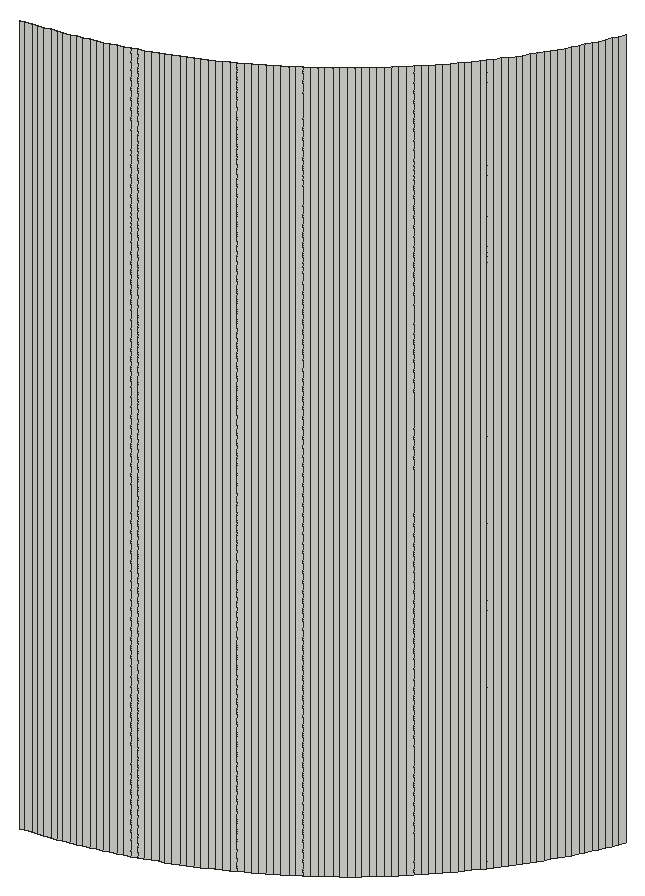
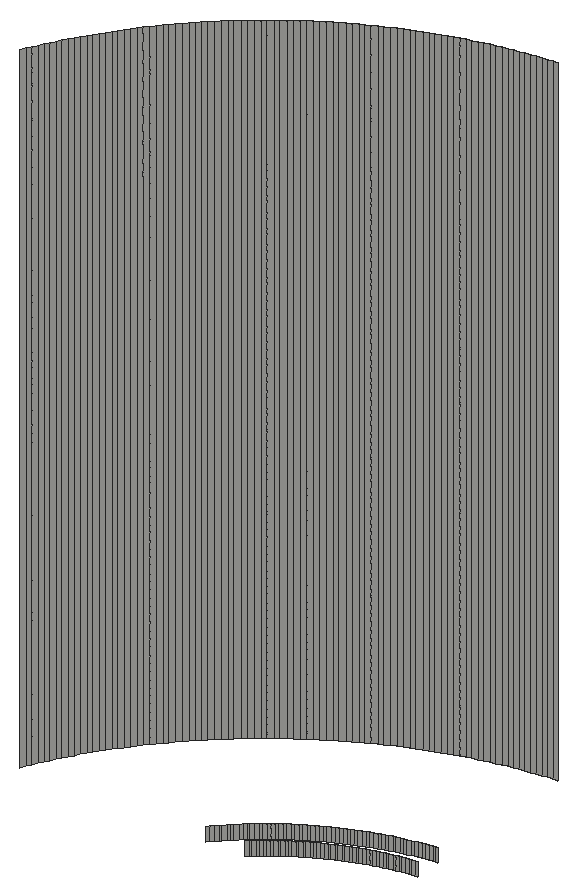
# SketchUp Ruby script. Lengths in inches.
U = 1.inch
M = Sketchup.active_model
def pt(a) = Geom::Point3d.new(a.map { |v| v * U })
def face(e, loops, mat)
  f = e.add_face(loops[0].map { |a| pt(a) })
  loops[1..].each { |l| e.add_face(l.map { |a| pt(a) }).erase! }
  f.material = f.back_material = mat if mat
  f
end
# faces: each face lists its corners as indices into pts; further lists are holes
def faces(e, pts, list, mat = nil) = list.each { |f| face(e, (f[0].is_a?(Array) ? f : [f]).map { |l| l.map { |i| pts[i] } }, mat) }
# xy, xz, yz: faces in a plane at the given z, y or x. An outline is a flat list of corners, or four numbers for a rectangle; further outlines are holes
def ring(l) = l.size == 4 ? [[l[0], l[1]], [l[2], l[1]], [l[2], l[3]], [l[0], l[3]]] : l.each_slice(2).to_a
def flat(e, list, mat, &to3) = list.each { |f| face(e, (f[0].is_a?(Array) ? f : [f]).map { |l| ring(l).map { |u, v| to3.(u, v) } }, mat) }
def xy(e, z, list, mat = nil) = flat(e, list, mat) { |x, y| [x, y, z] }
def xz(e, y, list, mat = nil) = flat(e, list, mat) { |x, z| [x, y, z] }
def yz(e, x, list, mat = nil) = flat(e, list, mat) { |y, z| [x, y, z] }
def lines(e, pts, list) = list.each { |a, b| e.add_line(pt(pts[a]), pt(pts[b])) }
# prism: a flat outline (further loops are holes) pulled along v
def prism(e, loops, v, mat = nil)
  f = face(e, loops, mat); d = Geom::Vector3d.new(v.map { |x| x * U })
  f.pushpull(f.normal.samedirection?(d) ? d.length : -d.length)
end
def box(e, o, s, mat = nil) = prism(e, [[o, [o[0] + s[0], o[1], o[2]], [o[0] + s[0], o[1] + s[1], o[2]], [o[0], o[1] + s[1], o[2]]]], [0, 0, s[2]], mat)
def at(x, y, z, deg = 0) = Geom::Transformation.translation(pt([x, y, z])) * Geom::Transformation.rotation(ORIGIN, Z_AXIS, deg.degrees)
def axes(o, x, y, z) = Geom::Transformation.new([*x, 0, *y, 0, *z, 0, *pt(o).to_a, 1])
def part(name) = M.definitions.add(name)
# library, detail: a bought-in or finely detailed component or shape, given as its bounding box
def library(name, o, s) = part(name).tap { |d| box(d.entities, o, s) }
def detail(e, o, s) = box(e.add_group.entities, o, s)
def put(e, d, t, mat = nil) = e.add_instance(d, t).tap { |i| i.material = mat if mat }
def group(e, t, mat = nil) = e.add_group.tap { |g| g.transformation = t; g.material = mat if mat }.entities
root = M.entities
p = [[368.95,214,228],[369.1,214.01,228],[369.1,214.01,252],[368.95,214,252],[369.29,214.04,228],[369.29,214.04,252],
  [369.48,214.0625,228],[369.48,214.0625,252],[369.67,214.09,228],[369.67,214.09,252],[369.85,214.12,228],[369.85,214.12,252],
  [370.04,214.15,228],[370.04,214.15,252],[370.23,214.18,228],[370.23,214.18,252],[370.42,214.22,228],[370.42,214.22,252],
  [370.61,214.25,228],[370.61,214.25,252],[370.8,214.29,228],[370.8,214.29,252],[370.98,214.34,228],[370.98,214.34,252],
  [371.17,214.38,228],[371.17,214.38,252],[371.35,214.43,228],[371.35,214.43,252],[371.54,214.48,228],[371.54,214.48,252],
  [371.72,214.53,228],[371.72,214.53,252],[371.91,214.58,228],[371.91,214.58,252],[372.09,214.64,228],[372.09,214.64,252],
  [372.27,214.7,228],[372.27,214.7,252],[372.45,214.76,228],[372.45,214.76,252],[372.64,214.82,228],[372.64,214.82,252],
  [372.82,214.89,228],[372.82,214.89,252],[372.99,214.95,228],[372.99,214.95,252],[373.17,215.02,228],[373.17,215.02,252],
  [373.35,215.1,228],[373.35,215.1,252],[373.53,215.17,228],[373.53,215.17,252],[373.7,215.25,228],[373.7,215.25,252],
  [373.88,215.32,228],[373.88,215.32,252],[374.05,215.41,228],[374.05,215.41,252],[374.22,215.49,228],[374.22,215.49,252],
  [374.4,215.57,228],[374.4,215.57,252],[374.57,215.66,228],[374.57,215.66,252],[374.74,215.75,228],[374.74,215.75,252],
  [374.91,215.84,228],[374.91,215.84,252],[375.07,215.93,228],[375.07,215.93,252],[375.24,216.03,228],[375.24,216.03,252],
  [375.4,216.125,228],[375.4,216.125,252],[375.57,216.22,228],[375.57,216.22,252],[375.73,216.32,228],[375.73,216.32,252],
  [375.89,216.43,228],[375.89,216.43,252],[376.05,216.53,228],[376.05,216.53,252],[376.21,216.64,228],[376.21,216.64,252],
  [376.37,216.75,228],[376.37,216.75,252],[376.52,216.86,228],[376.52,216.86,252],[376.68,216.97,228],[376.68,216.97,252],
  [376.83,217.09,228],[376.83,217.09,252],[376.98,217.2,228],[376.98,217.2,252],[377.13,217.32,228],[377.13,217.32,252],
  [377.28,217.44,228],[377.28,217.44,252],[377.43,217.56,228],[377.43,217.56,252],[377.58,217.6875,228],[377.58,217.6875,252],
  [377.72,217.8125,228],[377.72,217.8125,252],[377.86,217.94,228],[377.86,217.94,252],[378.01,218.07,228],[378.01,218.07,252],
  [378.15,218.2,228],[378.15,218.2,252],[378.28,218.33,228],[378.28,218.33,252],[378.42,218.47,228],[378.42,218.47,252],
  [378.56,218.61,228],[378.56,218.61,252],[378.6875,218.74,228],[378.6875,218.74,252],[378.82,218.88,228],[378.82,218.88,252],
  [378.95,219.02,228],[378.95,219.02,252],[379.08,219.17,228],[379.08,219.17,252],[379.2,219.31,228],[379.2,219.31,252],
  [379.33,219.46,228],[379.33,219.46,252],[379.45,219.6,228],[379.45,219.6,252],[379.57,219.75,228],[379.57,219.75,252],
  [379.69,219.9,228],[379.69,219.9,252],[379.81,220.05,228],[379.81,220.05,252],[368.6875,220.01,228],[368.62,220,228],
  [368.62,220,228.5],[368.6875,220.01,228.5],[368.8,220.02,228],[368.8,220.02,228.5],[368.92,220.04,228],[368.92,220.04,228.5],
  [369.03,220.0625,228],[369.03,220.0625,228.5],[369.15,220.08,228],[369.15,220.08,228.5],[369.27,220.1,228],[369.27,220.1,228.5],
  [369.38,220.13,228],[369.38,220.13,228.5],[369.5,220.15,228],[369.5,220.15,228.5],[379.92,220.21,228],[379.92,220.21,252],
  [369.61,220.18,228],[369.61,220.18,228.5],[369.73,220.21,228],[369.73,220.21,228.5],[369.84,220.23,228],[369.84,220.23,228.5],
  [369.95,220.27,228],[369.95,220.27,228.5],[380.04,220.36,228],[380.04,220.36,252],[370.07,220.3,228],[370.07,220.3,228.5],
  [370.18,220.33,228],[370.18,220.33,228.5],[370.29,220.36,228],[370.29,220.36,228.5],[370.41,220.4,228],[370.41,220.4,228.5],
  [370.52,220.4375,228],[370.52,220.4375,228.5],[370.63,220.48,228],[370.63,220.48,228.5],[380.15,220.52,228],[380.15,220.52,252],
  [370.74,220.52,228],[370.74,220.52,228.5],[370.85,220.56,228],[370.85,220.56,228.5],[380.26,220.67,228],[380.26,220.67,252],
  [370.96,220.6,228],[370.96,220.6,228.5],[371.07,220.65,228],[371.07,220.65,228.5],[371.18,220.69,228],[371.18,220.69,228.5],
  [371.28,220.74,228],[371.28,220.74,228.5],[371.39,220.79,228],[371.39,220.79,228.5],[380.36,220.83,228],[380.36,220.83,252],
  [371.5,220.84,228],[371.5,220.84,228.5],[371.61,220.89,228],[371.61,220.89,228.5],[380.47,220.99,228],[380.47,220.99,252],
  [371.71,220.9375,228],[371.71,220.9375,228.5],[371.82,220.99,228],[371.82,220.99,228.5],[368.56,221,228],[368.66,221.01,228],
  [368.66,221.01,228.5],[368.56,221,228.5],[368.76,221.03,228],[368.76,221.03,228.5],[368.87,221.05,228],[368.87,221.05,228.5],
  [368.97,221.07,228],[368.97,221.07,228.5],[371.92,221.05,228],[371.92,221.05,228.5],[372.02,221.1,228],[372.02,221.1,228.5],
  [380.57,221.15,228],[380.57,221.15,252],[369.07,221.09,228],[369.07,221.09,228.5],[369.18,221.11,228],[369.18,221.11,228.5],
  [369.28,221.13,228],[369.28,221.13,228.5],[369.38,221.15,228],[369.38,221.15,228.5],[372.125,221.16,228],[372.125,221.16,228.5],
  [369.49,221.18,228],[369.49,221.18,228.5],[369.59,221.2,228],[369.59,221.2,228.5],[369.69,221.23,228],[369.69,221.23,228.5],
  [369.79,221.26,228],[369.79,221.26,228.5],[372.23,221.22,228],[372.23,221.22,228.5],[372.33,221.28,228],[372.33,221.28,228.5],
  [380.68,221.31,228],[380.68,221.31,252],[369.89,221.29,228],[369.89,221.29,228.5],[369.99,221.32,228],[369.99,221.32,228.5],
  [370.09,221.35,228],[370.09,221.35,228.5],[372.43,221.34,228],[372.43,221.34,228.5],[372.53,221.4,228],[372.53,221.4,228.5],
  [380.78,221.48,228],[380.78,221.48,252],[370.19,221.38,228],[370.19,221.38,228.5],[370.29,221.42,228],[370.29,221.42,228.5],
  [370.39,221.46,228],[370.39,221.46,228.5],[372.63,221.46,228],[372.63,221.46,228.5],[370.49,221.49,228],[370.49,221.49,228.5],
  [370.59,221.53,228],[370.59,221.53,228.5],[370.6875,221.57,228],[370.6875,221.57,228.5],[372.73,221.53,228],[372.73,221.53,228.5],
  [372.83,221.59,228],[372.83,221.59,228.5],[380.87,221.64,228],[380.87,221.64,252],[370.78,221.61,228],[370.78,221.61,228.5],
  [370.88,221.65,228],[370.88,221.65,228.5],[372.92,221.66,228],[372.92,221.66,228.5],[380.97,221.81,228],[380.97,221.81,252],
  [370.98,221.7,228],[370.98,221.7,228.5],[371.07,221.74,228],[371.07,221.74,228.5],[371.17,221.79,228],[371.17,221.79,228.5],
  [373.02,221.73,228],[373.02,221.73,228.5],[373.11,221.8,228],[373.11,221.8,228.5],[371.26,221.83,228],[371.26,221.83,228.5],
  [371.36,221.88,228],[371.36,221.88,228.5],[373.21,221.87,228],[373.21,221.87,228.5],[381.0625,221.98,228],[381.0625,221.98,252],
  [371.45,221.93,228],[371.45,221.93,228.5],[371.54,221.98,228],[371.54,221.98,228.5],[373.3,221.94,228],[373.3,221.94,228.5],
  [373.39,222.01,228],[373.39,222.01,228.5],[371.64,222.03,228],[371.64,222.03,228.5],[371.73,222.08,228],[371.73,222.08,228.5],
  [373.49,222.09,228],[373.49,222.09,228.5],[381.15,222.14,228],[381.15,222.14,252],[371.82,222.14,228],[371.82,222.14,228.5],
  [371.91,222.19,228],[371.91,222.19,228.5],[373.58,222.16,228],[373.58,222.16,228.5],[381.24,222.3125,228],[381.24,222.3125,252],
  [372,222.25,228],[372,222.25,228.5],[372.09,222.3,228],[372.09,222.3,228.5],[373.67,222.24,228],[373.67,222.24,228.5],
  [373.76,222.32,228],[373.76,222.32,228.5],[372.17,222.36,228],[372.17,222.36,228.5],[373.84,222.39,228],[373.84,222.39,228.5],
  [381.33,222.48,228],[381.33,222.48,252],[372.26,222.42,228],[372.26,222.42,228.5],[372.35,222.48,228],[372.35,222.48,228.5],
  [373.93,222.47,228],[373.93,222.47,228.5],[372.43,222.54,228],[372.43,222.54,228.5],[372.52,222.6,228],[372.52,222.6,228.5],
  [374.02,222.55,228],[374.02,222.55,228.5],[381.42,222.66,228],[381.42,222.66,252],[372.6,222.67,228],[372.6,222.67,228.5],
  [374.1,222.64,228],[374.1,222.64,228.5],[374.18,222.72,228],[374.18,222.72,228.5],[372.6875,222.73,228],[372.6875,222.73,228.5],
  [372.77,222.8,228],[372.77,222.8,228.5],[374.27,222.8,228],[374.27,222.8,228.5],[381.5,222.83,228],[381.5,222.83,252],
  [372.85,222.86,228],[372.85,222.86,228.5],[374.35,222.89,228],[374.35,222.89,228.5],[381.58,223,228],[381.58,223,252],
  [372.93,222.93,228],[372.93,222.93,228.5],[373.01,223,228],[373.01,223,228.5],[374.43,222.97,228],[374.43,222.97,228.5],
  [373.09,223.07,228],[373.09,223.07,228.5],[374.51,223.06,228],[374.51,223.06,228.5],[381.66,223.18,228],[381.66,223.18,252],
  [373.17,223.14,228],[373.17,223.14,228.5],[373.25,223.21,228],[373.25,223.21,228.5],[374.59,223.15,228],[374.59,223.15,228.5],
  [374.67,223.24,228],[374.67,223.24,228.5]]
faces(root,p,[[0,1,2,3],[1,4,5,2],[4,6,7,5],[6,8,9,7],[8,10,11,9],[10,12,13,11],[12,14,15,13],[14,16,17,15],
  [16,18,19,17],[18,20,21,19],[20,22,23,21],[22,24,25,23],[24,26,27,25],[26,28,29,27],[28,30,31,29],[30,32,33,31],
  [32,34,35,33],[34,36,37,35],[36,38,39,37],[38,40,41,39],[40,42,43,41],[42,44,45,43],[44,46,47,45],[46,48,49,47],
  [48,50,51,49],[50,52,53,51],[52,54,55,53],[54,56,57,55],[56,58,59,57],[58,60,61,59],[60,62,63,61],[62,64,65,63],
  [64,66,67,65],[66,68,69,67],[68,70,71,69],[70,72,73,71],[72,74,75,73],[74,76,77,75],[76,78,79,77],[78,80,81,79],
  [80,82,83,81],[82,84,85,83],[84,86,87,85],[86,88,89,87],[88,90,91,89],[90,92,93,91],[92,94,95,93],[94,96,97,95],
  [96,98,99,97],[98,100,101,99],[100,102,103,101],[102,104,105,103],[104,106,107,105],[106,108,109,107],[108,110,111,109],[110,112,113,111],
  [112,114,115,113],[114,116,117,115],[116,118,119,117],[118,120,121,119],[120,122,123,121],[122,124,125,123],[124,126,127,125],[126,128,129,127],
  [128,130,131,129],[130,132,133,131],[132,134,135,133],[136,137,138,139],[140,136,139,141],[142,140,141,143],[144,142,143,145],[146,144,145,147],
  [148,146,147,149],[150,148,149,151],[152,150,151,153],[134,154,155,135],[156,152,153,157],[158,156,157,159],[160,158,159,161],[162,160,161,163],
  [154,164,165,155],[166,162,163,167],[168,166,167,169],[170,168,169,171],[172,170,171,173],[174,172,173,175],[176,174,175,177],[164,178,179,165],
  [180,176,177,181],[182,180,181,183],[178,184,185,179],[186,182,183,187],[188,186,187,189],[190,188,189,191],[192,190,191,193],[194,192,193,195],
  [184,196,197,185],[198,194,195,199],[200,198,199,201],[196,202,203,197],[204,200,201,205],[206,204,205,207],[208,209,210,211],[209,212,213,210],
  [212,214,215,213],[214,216,217,215],[218,206,207,219],[220,218,219,221],[202,222,223,203],[216,224,225,217],[224,226,227,225],[226,228,229,227],
  [228,230,231,229],[232,220,221,233],[230,234,235,231],[234,236,237,235],[236,238,239,237],[238,240,241,239],[242,232,233,243],[244,242,243,245],
  [222,246,247,223],[240,248,249,241],[248,250,251,249],[250,252,253,251],[254,244,245,255],[256,254,255,257],[246,258,259,247],[252,260,261,253],
  [260,262,263,261],[262,264,265,263],[266,256,257,267],[264,268,269,265],[268,270,271,269],[270,272,273,271],[274,266,267,275],[276,274,275,277],
  [258,278,279,259],[272,280,281,273],[280,282,283,281],[284,276,277,285],[278,286,287,279],[282,288,289,283],[288,290,291,289],[290,292,293,291],
  [294,284,285,295],[296,294,295,297],[292,298,299,293],[298,300,301,299],[302,296,297,303],[286,304,305,287],[300,306,307,301],[306,308,309,307],
  [310,302,303,311],[312,310,311,313],[308,314,315,309],[314,316,317,315],[318,312,313,319],[304,320,321,305],[316,322,323,317],[322,324,325,323],
  [326,318,319,327],[320,328,329,321],[324,330,331,325],[330,332,333,331],[334,326,327,335],[336,334,335,337],[332,338,339,333],[340,336,337,341],
  [328,342,343,329],[338,344,345,339],[344,346,347,345],[348,340,341,349],[346,350,351,347],[350,352,353,351],[354,348,349,355],[342,356,357,343],
  [352,358,359,353],[360,354,355,361],[362,360,361,363],[358,364,365,359],[364,366,367,365],[368,362,363,369],[356,370,371,357],[366,372,373,367],
  [374,368,369,375],[370,376,377,371],[372,378,379,373],[378,380,381,379],[382,374,375,383],[380,384,385,381],[386,382,383,387],[376,388,389,377],
  [384,390,391,385],[390,392,393,391],[394,386,387,395],[396,394,395,397]])
